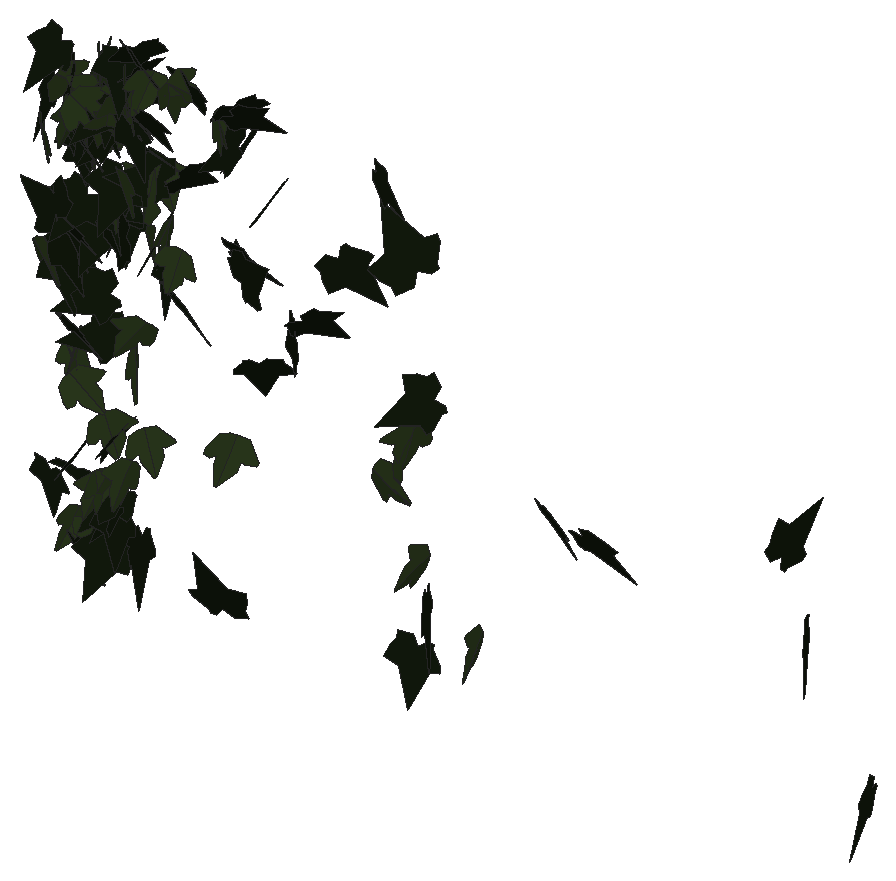
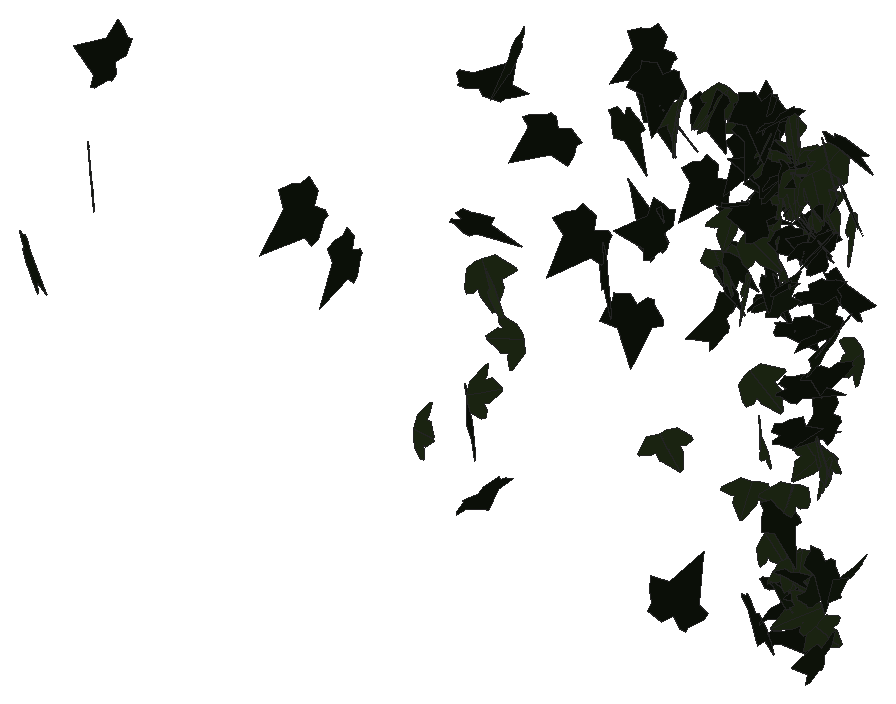
# SketchUp Ruby script. Lengths in inches.
U = 1.inch
M = Sketchup.active_model
def pt(a) = Geom::Point3d.new(a.map { |v| v * U })
def face(e, loops, mat)
  f = e.add_face(loops[0].map { |a| pt(a) })
  loops[1..].each { |l| e.add_face(l.map { |a| pt(a) }).erase! }
  f.material = f.back_material = mat if mat
  f
end
# faces: each face lists its corners as indices into pts; further lists are holes
def faces(e, pts, list, mat = nil) = list.each { |f| face(e, (f[0].is_a?(Array) ? f : [f]).map { |l| l.map { |i| pts[i] } }, mat) }
# xy, xz, yz: faces in a plane at the given z, y or x. An outline is a flat list of corners, or four numbers for a rectangle; further outlines are holes
def ring(l) = l.size == 4 ? [[l[0], l[1]], [l[2], l[1]], [l[2], l[3]], [l[0], l[3]]] : l.each_slice(2).to_a
def flat(e, list, mat, &to3) = list.each { |f| face(e, (f[0].is_a?(Array) ? f : [f]).map { |l| ring(l).map { |u, v| to3.(u, v) } }, mat) }
def xy(e, z, list, mat = nil) = flat(e, list, mat) { |x, y| [x, y, z] }
def xz(e, y, list, mat = nil) = flat(e, list, mat) { |x, z| [x, y, z] }
def yz(e, x, list, mat = nil) = flat(e, list, mat) { |y, z| [x, y, z] }
def lines(e, pts, list) = list.each { |a, b| e.add_line(pt(pts[a]), pt(pts[b])) }
# prism: a flat outline (further loops are holes) pulled along v
def prism(e, loops, v, mat = nil)
  f = face(e, loops, mat); d = Geom::Vector3d.new(v.map { |x| x * U })
  f.pushpull(f.normal.samedirection?(d) ? d.length : -d.length)
end
def box(e, o, s, mat = nil) = prism(e, [[o, [o[0] + s[0], o[1], o[2]], [o[0] + s[0], o[1] + s[1], o[2]], [o[0], o[1] + s[1], o[2]]]], [0, 0, s[2]], mat)
def at(x, y, z, deg = 0) = Geom::Transformation.translation(pt([x, y, z])) * Geom::Transformation.rotation(ORIGIN, Z_AXIS, deg.degrees)
def axes(o, x, y, z) = Geom::Transformation.new([*x, 0, *y, 0, *z, 0, *pt(o).to_a, 1])
def part(name) = M.definitions.add(name)
# library, detail: a bought-in or finely detailed component or shape, given as its bounding box
def library(name, o, s) = part(name).tap { |d| box(d.entities, o, s) }
def detail(e, o, s) = box(e.add_group.entities, o, s)
def put(e, d, t, mat = nil) = e.add_instance(d, t).tap { |i| i.material = mat if mat }
def group(e, t, mat = nil) = e.add_group.tap { |g| g.transformation = t; g.material = mat if mat }.entities
root = M.entities
M.materials.add("efeu1").color = [18, 25, 13]
M.materials.add("efeu2").color = [43, 57, 29]
c1 = part("ivyleaf_9")
p = [[1.54,2.16,1.25],[1.36,2.04,1.19],[-0.21,0.99,0.68],[-0.71,1.11,0.82],[-0.85,0.86,0.67],[-0.8,0.17,0.21],
  [-0.9,-0.01,0.1],[-0.67,-0.16,-0.02],[-0.08,-0.08,-0.05],[-0.03,-0.6,-0.4],[0.65,-0.88,-0.66],[0.83,-0.6,-0.49],
  [1.29,-0.42,-0.43],[1.8125,-0.07,-0.26],[1.21,0.44,0.15]]
faces(c1.entities,p,[[0,1,2,3,4,5,6,7,8,9,10,11,12,13,14]],"efeu1")
c2 = part("ivyleaf_10")
p = [[0,0.5,-0.03],[-0.0625,2.02,-0.43],[-0.19,2.01,-0.46],[-0.54,1.05,-0.29],[-0.52,0.625,-0.18],[-0.83,0.76,-0.28],
  [-1.16,0.64,-0.33],[-1.15,0.33,-0.24],[-0.77,-0.39,0.02],[-0.3,-0.51,0.16],[0.04,-0.48,0.23],[-0.02,2.01,-0.4375],
  [-0.06,2.01,-0.43],[0.04,-0.49,0.23],[0.67,-0.49,0.14],[1.38,0.36,-0.2],[1.375,0.51,-0.24],[0.81,0.65,-0.19],
  [0.62,0.59,-0.15],[0.6,1.09,-0.28],[0.5,1.23,-0.31]]
faces(c2.entities,p,[[0,1,2,3,4,5,6,7,8,9,10],[11,12,0,13,14,15,16,17,18,19,20]],"efeu2")
put(root,c1,axes([597.28,127.56,272.27],[-0.86888,0.24812,-0.71186],[0.69463,-0.15856,-0.90312],[-0.29292,-1.11201,-0.03006]))
put(root,c2,axes([597.45,126.56,269.88],[-0.79765,0.80045,0.26737],[-0.26507,0.11165,-1.12504],[-0.80122,-0.83382,0.10602]))
put(root,c2,axes([596.9,127.04,262.04],[-0.78007,0.51311,-0.68013],[0.58115,-0.35385,-0.9335],[-0.623,-0.97256,-0.01919]))
put(root,c1,axes([598.54,126.26,264.96],[-0.28298,0.30456,1.14676],[-0.84466,0.77623,-0.41459],[-0.83327,-0.89027,0.03081]))
put(root,c1,axes([598.08,127.12,275.29],[-1.11568,-0.20178,-0.20387],[0.21416,-0.04129,-1.13112],[0.19082,-1.1334,0.0775]))
put(root,c1,axes([597.28,127.38,247.86],[0.15901,-0.96979,0.43911],[0.1888,-0.41125,-0.97664],[1.04769,0.2213,0.10935]))
put(root,c1,axes([598.375,127.92,248.8],[-0.16339,1.01209,0.32974],[-0.03918,0.32766,-1.02511],[-1.06373,-0.16753,-0.01289]))
put(root,c2,axes([597.93,128.29,255.16],[-0.69515,0.83202,-0.14465],[0.08789,-0.11506,-1.08418],[-0.83992,-0.70066,0.00627]))
put(root,c1,axes([597.46,129.11,262.94],[0.46202,-0.94385,0.29757],[0.12279,-0.27119,-1.05083],[0.982,0.47798,-0.0086]))
put(root,c2,axes([598.27,128.4375,244.87],[0.3494,0.74419,-0.66645],[-0.31055,-0.59015,-0.82179],[-0.94949,0.46687,0.02354]))
put(root,c1,axes([597.68,129.15,247.42],[-0.25311,-0.81514,0.53357],[0.7054,-0.53358,-0.48054],[0.67199,0.25308,0.70541]))
put(root,c1,axes([597.91,128.09,261.29],[-0.25288,-0.98758,-0.43939],[0.21656,0.39581,-1.01428],[1.059,-0.31677,0.10249]))
put(root,c2,axes([598.38,127.83,254.61],[0.76201,-0.89613,0.14041],[-0.09117,0.10679,1.17631],[-0.90247,-0.76745,-0.00027]))
put(root,c1,axes([598.11,128.9,269.02],[0.2264,-1.07078,0.10416],[0.02246,-0.10172,-1.09445],[1.0756,0.22751,0.00093]))
put(root,c1,axes([599.3125,127.72,268.87],[-0.13512,0.56337,0.94543],[-0.62323,0.74591,-0.53355],[-0.90709,-0.59641,0.22576]))
put(root,c1,axes([597.9,128.74,243.47],[0.79455,-0.80897,0.29888],[0.2054,-0.21719,-1.1339],[0.8376,0.82066,-0.00546]))
put(root,c2,axes([598.76,127.58,271.07],[-0.0654,-1.01073,0.46922],[0.05437,-0.47236,-1.00992],[1.11301,-0.03631,0.07691]))
put(root,c1,axes([598.49,128.91,269.4],[-0.16722,-1.05797,-0.24772],[-0.00201,0.25094,-1.07035],[1.08658,-0.16235,-0.04011]))
put(root,c2,axes([598.96,128.1,272.65],[-0.38508,-1.04047,0.20579],[0.00633,-0.22118,-1.10646],[1.0606,-0.37645,0.08132]))
put(root,c1,axes([598.36,126.99,262.92],[0.55398,-0.95704,-0.25403],[-0.11777,0.22533,-1.10576],[0.98315,0.56626,0.01068]))
put(root,c2,axes([598.6,127.84,255.63],[1.06122,-0.21206,0.17514],[0.1743,-0.02144,-1.08213],[0.21275,1.07536,0.01296]))
put(root,c1,axes([597.95,128.51,268.79],[0.62885,-0.44126,0.80937],[0.6514,-0.48056,-0.76811],[0.65228,0.90532,-0.01323]))
put(root,c1,axes([598.41,127.17,264.08],[1.07583,-0.17845,-0.0565],[-0.05514,0.01285,-1.09052],[0.17887,1.07723,0.00365]))
put(root,c1,axes([598.61,127.42,274.03],[-0.52514,0.03385,-1.03029],[1.0051,-0.23997,-0.52018],[-0.22893,-1.13123,0.07952]))
put(root,c1,axes([598.46,127.24,257.83],[1.07839,-0.24368,-0.01207],[-0.01122,0.0051,-1.10558],[0.24372,1.07845,0.0025]))
put(root,c1,axes([599.29,127.96,265.7],[-0.71522,-0.82021,0.27547],[-0.18549,-0.20373,-1.08823],[0.84511,-0.73886,-0.00573]))
put(root,c2,axes([598.86,126.63,273.66],[-0.46528,-0.6187,-0.89971],[0.58288,0.68625,-0.77334],[0.92332,-0.745,0.03482]))
put(root,c1,axes([598.8,127.29,270.21],[0.7809,-0.6817,0.42925],[0.3105,-0.29694,-1.03643],[0.74335,0.84017,-0.01802]))
put(root,c1,axes([600.27,128.68,259.5],[-0.78658,-0.32714,0.70864],[-0.64347,-0.29759,-0.85163],[0.44173,-1.01603,0.02127]))
put(root,c2,axes([599.625,127.7,269.31],[-0.66455,0.88841,0.028],[-0.01312,0.02515,-1.10945],[-0.88875,-0.66467,-0.00456]))
put(root,c1,axes([600.34,129.1,256.73],[-0.6642,-0.21197,0.84357],[-0.75872,-0.3778,-0.69232],[0.42531,-1.00501,0.08234]))
put(root,c2,axes([600.13,127.48,273.01],[-0.37141,-0.62185,0.894],[-0.36383,-0.81944,-0.72113],[1.02643,-0.51547,0.06788]))
put(root,c1,axes([600.29,127.47,273.08],[-0.10286,1.06931,-0.33204],[-0.26852,-0.34727,-1.03516],[-1.08701,-0.0154,0.28714]))
put(root,c1,axes([599.88,128.82,263.76],[-0.77813,-0.76443,-0.08932],[0.04636,0.08024,-1.09051],[0.76823,-0.77911,-0.02467]))
put(root,c2,axes([599.39,127.86,245.37],[0.24919,0.22073,1.11663],[0.43673,1.03704,-0.30246],[-1.05111,0.48322,0.13905]))
put(root,c2,axes([600.14,128.26,272.66],[-0.35087,-1.06359,-0.0843],[0.0119,0.08483,-1.11987],[1.06686,-0.35074,-0.01523]))
put(root,c2,axes([600.25,128.53,272.44],[-1.08179,0.25748,0.11079],[-0.15217,-0.16852,-1.09421],[-0.23541,-1.07431,0.1982]))
put(root,c2,axes([599.62,126.73,254.62],[0.5894,0.63968,0.77751],[0.56026,0.54019,-0.86914],[-0.83655,0.81247,-0.03428]))
put(root,c2,axes([600.42,128.01,247.98],[-0.37474,-0.93259,0.60477],[0.00705,-0.6402,-0.98286],[1.1115,-0.31036,0.21014]))
put(root,c2,axes([600.48,128.14,248.13],[0.36073,1.09946,-0.18153],[-0.21386,-0.11895,-1.14543],[-1.09363,0.38592,0.16411]))
put(root,c2,axes([600.83,127.41,275.125],[-0.80917,0.71764,0.32519],[-0.40581,0.01994,-1.05377],[-0.67534,-0.87184,0.24357]))
put(root,c1,axes([600.72,128.35,243.79],[-0.76762,-0.84848,-0.00863],[0.00333,0.00863,-1.14418],[0.84852,-0.76762,-0.00332]))
put(root,c1,axes([600.07,127.91,271.82],[0.66739,-0.89287,0.00332],[0.00202,-0.00264,-1.11473],[0.89288,0.66739,0.00004]))
put(root,c2,axes([600.28,126.01,272.77],[0.47672,0.80066,0.82643],[0.26344,0.79484,-0.92203],[-1.12011,0.5277,0.13488]))
put(root,c2,axes([600.77,127.82,275.38],[0.32811,-1.08627,-0.10958],[0.00978,0.11734,-1.13392],[1.09174,0.32542,0.04309]))
put(root,c1,axes([601.06,128.78,247.3],[-0.93964,-0.56298,0.2136],[-0.15344,-0.15895,-1.09393],[0.58226,-0.95041,0.05643]))
put(root,c1,axes([601.3,128.34,246.53],[-0.97263,0.57833,-0.25387],[0.20544,-0.15111,-1.13131],[-0.59725,-0.99379,0.02428]))
put(root,c1,axes([601.22,127.98,272.06],[-0.9302,-0.55,0.25967],[-0.10674,-0.3195,-1.05911],[0.59878,-0.91138,0.21459]))
put(root,c1,axes([601.37,128.21,251.17],[-0.39112,1.05139,-0.17096],[0.05988,-0.16014,-1.12178],[-1.06352,-0.39567,-0.00028]))
put(root,c1,axes([600.75,128.38,272.6875],[-0.2683,-1.0801,-0.10082],[0.0306,0.09628,-1.11291],[1.08436,-0.26996,0.00646]))
put(root,c1,axes([601.57,127.26,270.64],[-0.97691,0.52652,-0.06574],[0.05706,-0.03268,-1.10976],[-0.52753,-0.97857,0.00169]))
put(root,c2,axes([601.13,127.04,271.59],[-1.08266,-0.24176,-0.06386],[0.06414,0.00577,-1.1093],[0.24169,-1.08453,0.00833]))
put(root,c1,axes([601.19,129.4,264.59],[-0.85276,-0.49925,0.47095],[0.32313,-0.95473,-0.427],[0.6055,-0.19362,0.89114]))
put(root,c1,axes([600.88,128.72,245.68],[0.02081,-1.10274,0.10467],[0.00514,-0.10459,-1.10293],[1.10768,0.0212,0.00315]))
put(root,c2,axes([601.52,127.41,271.59],[-0.32064,-1.03118,0.231],[-0.10634,-0.20869,-1.07918],[1.05137,-0.33559,-0.0387]))
put(root,c2,axes([601.07,127.59,252.16],[0.70534,0.84982,0.3555],[0.05352,0.40917,-1.08434],[-0.91963,0.67562,0.20955]))
put(root,c1,axes([601.95,128.51,265.71],[-0.70349,0.54739,-0.66374],[0.54603,-0.37849,-0.89089],[-0.66485,-0.89005,-0.02936]))
put(root,c1,axes([601.46,128.78,265.06],[-0.09904,-1.09832,-0.04645],[0.09129,0.03826,-1.0993],[1.0955,-0.10248,0.08741]))
put(root,c2,axes([601.64,128.37,273.55],[1.10422,0.10414,0.03894],[0.03821,0.0096,-1.1091],[-0.10441,1.10486,0.00596]))
put(root,c1,axes([602.64,127.24,264.56],[-0.16451,0.03207,-1.14396],[-1.14398,-0.03628,0.1635],[-0.03136,1.15516,0.03689]))
put(root,c2,axes([601.78,128.06,271.73],[1.04114,-0.37727,-0.00631],[0.06243,0.19051,-1.08911],[0.37212,1.02358,0.20038]))
put(root,c2,axes([601.43,127.99,266.74],[0.76668,-0.48593,0.67987],[0.5963,-0.32829,-0.90708],[0.58547,0.97069,0.03357]))
put(root,c1,axes([601,128.55,272.54],[0.53082,-0.13605,0.96901],[0.93611,-0.25041,-0.54796],[0.28494,1.07613,-0.005]))
put(root,c1,axes([601.17,128.52,272.44],[0.77239,-0.70065,0.39286],[0.3359,-0.21336,-1.0409],[0.72967,0.83988,0.06331]))
put(root,c2,axes([602.03,128.33,273.54],[-0.41694,-0.94867,0.42173],[0.1085,-0.49179,-0.99901],[1.0325,-0.33141,0.27528]))
put(root,c2,axes([601.95,128.28,249.12],[-0.26796,-0.91343,0.63261],[0.23456,-0.68259,-0.88624],[1.08607,-0.07794,0.34748]))
put(root,c2,axes([602.09,127.49,273.08],[-0.37328,-1.03666,-0.34856],[0.13341,0.32239,-1.10171],[1.08552,-0.3961,0.01554]))
put(root,c1,axes([602.21,127.6,267.9],[-0.64415,-0.99297,0.05727],[-0.03114,-0.04806,-1.18361],[0.99414,-0.6449,0.00004]))
put(root,c1,axes([602.02,127.76,275.3125],[-0.11588,-1.13441,-0.04033],[-0.01186,0.04175,-1.1402],[1.13506,-0.11538,-0.01603]))
put(root,c2,axes([603.11,128.48,267.65],[-0.55368,-0.26675,0.92514],[-0.83666,-0.39484,-0.61457],[0.47649,-1.00327,-0.00411]))
put(root,c2,axes([601.86,129.03,255.81],[0.74669,-0.57144,0.76372],[0.6868,-0.35094,-0.93407],[0.6619,1.00879,0.10766]))
put(root,c2,axes([602.3,127.93,274.36],[-0.28807,0.89779,-0.59532],[0.19145,-0.56376,-0.94283],[-1.06008,-0.34578,-0.0085]))
put(root,c1,axes([602.68,127.88,274.55],[0.31657,1.03061,0.29479],[0.06542,0.28823,-1.07792],[-1.06994,0.32256,0.02132]))
put(root,c1,axes([602.84,127.9,276.23],[0.29558,1.03464,-0.3641],[-0.11557,-0.34561,-1.07593],[-1.09073,0.317,0.01533]))
put(root,c2,axes([603.17,127.95,258.7],[-0.55276,-0.71768,0.69491],[-0.44298,-0.53575,-0.90567],[0.8954,-0.7081,-0.01907]))
put(root,c1,axes([602.44,128.95,244.625],[-0.7515,-0.08358,-1.09621],[1.09861,-0.00723,-0.7526],[0.04128,-1.32905,0.07303]))
put(root,c2,axes([602.84,126.77,268.56],[-0.85695,0.60816,-0.35576],[0.26248,-0.2443,-1.04987],[-0.65386,-0.89513,0.04482]))
put(root,c1,axes([602.17,128.55,269.43],[0.68165,-0.32808,0.8159],[0.75086,-0.32021,-0.75607],[0.45775,1.0138,0.02523]))
put(root,c1,axes([602.78,127.6,271.44],[0.39894,-1.03519,0.054],[0.03027,-0.0462,-1.10934],[1.03616,0.39992,0.01162]))
put(root,c1,axes([602.6875,127.96,275.5],[0.60417,-0.62119,0.73345],[0.51194,-0.52523,-0.86654],[0.81347,0.7919,0.0006]))
put(root,c2,axes([603.82,128.01,264.47],[-0.65847,0.85347,0.28196],[-0.22891,0.17878,-1.0757],[-0.8692,-0.69364,0.06969]))
put(root,c2,axes([603.51,128.02,251.8],[0.78708,0.74633,0.28902],[0.18704,0.2226,-1.0842],[-0.77818,0.80838,0.03172]))
put(root,c1,axes([604.71,127.89,268.55],[-0.75476,0.11676,0.82524],[-0.83345,-0.1122,-0.74639],[0.00484,-1.1127,0.16185]))
put(root,c2,axes([604.15,127.55,274.84],[0.73225,0.74241,-0.40554],[-0.42749,-0.1381,-1.0247],[-0.72999,0.82558,0.19327]))
put(root,c1,axes([604.02,127.03,272.8],[1.06564,0.19764,-0.26871],[-0.27281,-0.00121,-1.08278],[-0.19195,1.09899,0.04713]))
put(root,c2,axes([604.56,126.9,267.06],[0.91883,-0.66379,0.16953],[-0.13526,0.10228,1.13351],[-0.67161,-0.92873,0.00366]))
put(root,c2,axes([604.56,128.28,268.73],[0.3581,1.03504,0.25044],[-0.00111,0.26458,-1.09191],[-1.06491,0.34779,0.08535]))
put(root,c1,axes([605.1,127.87,265.91],[-0.75627,0.41017,-0.71675],[0.54703,-0.47925,-0.85146],[-0.61864,-0.92519,0.1233]))
put(root,c2,axes([605.02,128.06,265.63],[0.31295,-1.05852,0.16082],[0.21604,-0.10167,-1.08962],[1.04865,0.33684,0.17649]))
put(root,c1,axes([605.4375,127.7,263.98],[-0.72049,-0.06467,-0.89539],[0.89631,0.01255,-0.72213],[0.05033,-1.1492,0.0425]))
put(root,c1,axes([606.55,127.98,275.2],[0.28527,0.44154,-0.99676],[-1.00522,-0.29223,-0.41714],[-0.42193,0.99474,0.31989]))
put(root,c2,axes([606.09,127.27,274.76],[0.22805,-0.42079,-1.03271],[0.23097,1.04905,-0.37645],[1.09097,-0.13414,0.29557]))
put(root,c2,axes([605.98,127.36,275.3125],[-0.39804,-0.6389,-0.85217],[0.51801,0.67876,-0.75085],[0.93062,-0.65109,0.05346]))
put(root,c1,axes([605.45,127.9,261.7],[0.97644,-0.7129,0.23758],[0.19558,-0.13503,-1.20898],[0.72555,0.99582,0.00615]))
put(root,c2,axes([606.61,126.92,264.71],[1.1011,0.01348,-0.19923],[-0.19965,0.09441,-1.09705],[0.0036,1.11499,0.0953]))
put(root,c1,axes([606.72,127.15,269.79],[0.54844,0.8665,0.47006],[0.25016,0.39797,-1.02548],[-0.95352,0.6028,0.00133]))
put(root,c1,axes([608.27,128.78,242.57],[0.94497,-0.33268,0.91408],[-0.84147,0.35977,1.00085],[-0.48801,-1.26455,0.04426]))
put(root,c2,axes([608.83,127.95,273.2],[-0.78561,0.81372,0.11055],[-0.19647,-0.0377,-1.11872],[-0.79735,-0.79246,0.16674]))
put(root,c2,axes([608.94,127.73,273.95],[-0.20616,1.11368,-0.15147],[0.0171,-0.15088,-1.13255],[-1.1238,-0.2066,0.01055]))
put(root,c2,axes([609.18,128.56,253.1],[0.87695,0.72816,-0.40792],[-0.33046,-0.24042,-1.13959],[-0.76643,0.93682,0.02461]))
put(root,c1,axes([610.1,127.61,275.24],[0.42992,1.05413,-0.14889],[-0.06742,-0.1333,-1.13837],[-1.06246,0.43501,0.01198]))
put(root,c1,axes([610.67,127.05,273.125],[-0.98356,0.57281,0.12129],[-0.10474,0.06117,-1.1382],[-0.57607,-0.98912,-0.00015]))
put(root,c1,axes([611.08,127.33,273.21],[-0.66193,0.92991,-0.07281],[0.03972,-0.0611,-1.14144],[-0.93191,-0.66312,0.00307]))
put(root,c1,axes([609.79,128.04,265.72],[0.84755,-0.44388,0.65956],[0.61887,-0.23681,-0.95463],[0.49905,1.04751,0.06367]))
put(root,c1,axes([610.77,127.48,264.49],[-0.10045,0.08933,1.36953],[0.7557,-1.14268,0.12996],[1.14565,0.76157,0.03435]))
put(root,c1,axes([611.45,126.07,275.81],[0.94937,0.48409,0.42628],[0.36311,0.22583,-1.06514],[-0.53312,1.01588,0.03364]))
put(root,c1,axes([612.2,127.25,259.83],[0.61015,0.8973,-0.42177],[-0.28478,-0.31576,-1.08376],[-0.94971,0.67117,0.054]))
put(root,c1,axes([613.51,126.59,271.02],[-0.5711,1.00337,-0.11581],[0.06204,-0.09794,-1.1545],[-1.00812,-0.57443,-0.00544]))
put(root,c1,axes([614.39,127.49,262.22],[0.14858,0.01202,-1.22368],[-1.20978,0.18708,-0.14505],[0.18429,1.21839,0.03434]))
put(root,c1,axes([615.24,127.35,263.62],[0.89371,0.78416,0.33838],[0.23009,0.25059,-1.18844],[-0.82247,0.92218,0.03521]))
put(root,c1,axes([618.1875,126.86,268.73],[-0.1522,-0.23715,-1.21814],[0.66261,1.02216,-0.28179],[1.04931,-0.67987,0.00126]))
put(root,c1,axes([619.72,128.26,274.02],[0.88934,-0.54395,-0.59762],[-0.51603,0.30161,-1.04245],[0.62189,1.02815,-0.01037]))
put(root,c2,axes([620.16,128,255.32],[-0.42338,0.21866,-1.1022],[1.01436,-0.43238,-0.47542],[-0.48345,-1.0987,-0.03227]))
put(root,c2,axes([621.46,127.86,256.875],[0.54788,-0.86317,-0.64065],[0.45897,-0.46238,1.01549],[-0.97203,-0.70485,0.11839]))
put(root,c2,axes([622.43,127.83,258.82],[-0.60549,-1.0178,0.25521],[-0.1283,-0.22062,-1.18428],[1.04143,-0.61893,0.00248]))
put(root,c1,axes([623.16,127.19,269.83],[-1.30744,-0.60904,-0.07192],[-0.06386,-0.03323,1.44233],[-0.60994,1.30899,0.00315]))
put(root,c1,axes([622.33,128.41,244.98],[-0.18366,-1.20134,0.11107],[-0.00611,-0.11142,-1.21525],[1.20645,-0.18345,0.01076]))
put(root,c2,axes([622.93,127.98,250.87],[0.11763,-0.31093,1.16654],[0.28866,-1.13082,-0.33052],[1.17225,0.30966,-0.03567]))
put(root,c1,axes([623.84,127.8,261.45],[-1.11671,-0.15173,0.4622],[-0.45193,-0.10474,-1.12627],[0.18004,-1.20404,0.03972]))
put(root,c1,axes([623.86,127.33,248.97],[-0.30813,-0.04542,-1.39382],[1.36733,-0.29056,-0.29281],[-0.27425,-1.39759,0.10617]))
put(root,c2,axes([626.86,128.03,247.18],[0.25067,-0.66036,1.01602],[0.53732,-0.86938,-0.69762],[1.08613,0.58251,0.11063]))
put(root,c1,axes([631.58,128.21,256.91],[1.16227,-0.16369,-0.46715],[-0.46425,0.0532,-1.17369],[0.17175,1.25151,-0.01121]))
put(root,c1,axes([635.75,126.48,257.5],[1.39765,0.03322,0.01958],[0.0192,0.01629,-1.39796],[-0.03344,1.39769,0.01583]))
put(root,c1,axes([649.93,126.15,261.65],[-0.11455,-0.06879,1.32131],[0.81426,1.04169,0.12482],[-1.04287,0.8209,-0.04768]))
put(root,c1,axes([649.83,128.35,255.91],[-0.42186,0.13257,-1.2627],[1.21701,-0.3369,-0.44196],[-0.36176,-1.28797,-0.01436]))
put(root,c1,axes([655.37,127.05,248.07],[-0.89221,0.31655,-0.96952],[0.91156,-0.33024,-0.94669],[-0.45743,-1.27552,0.00449]))
